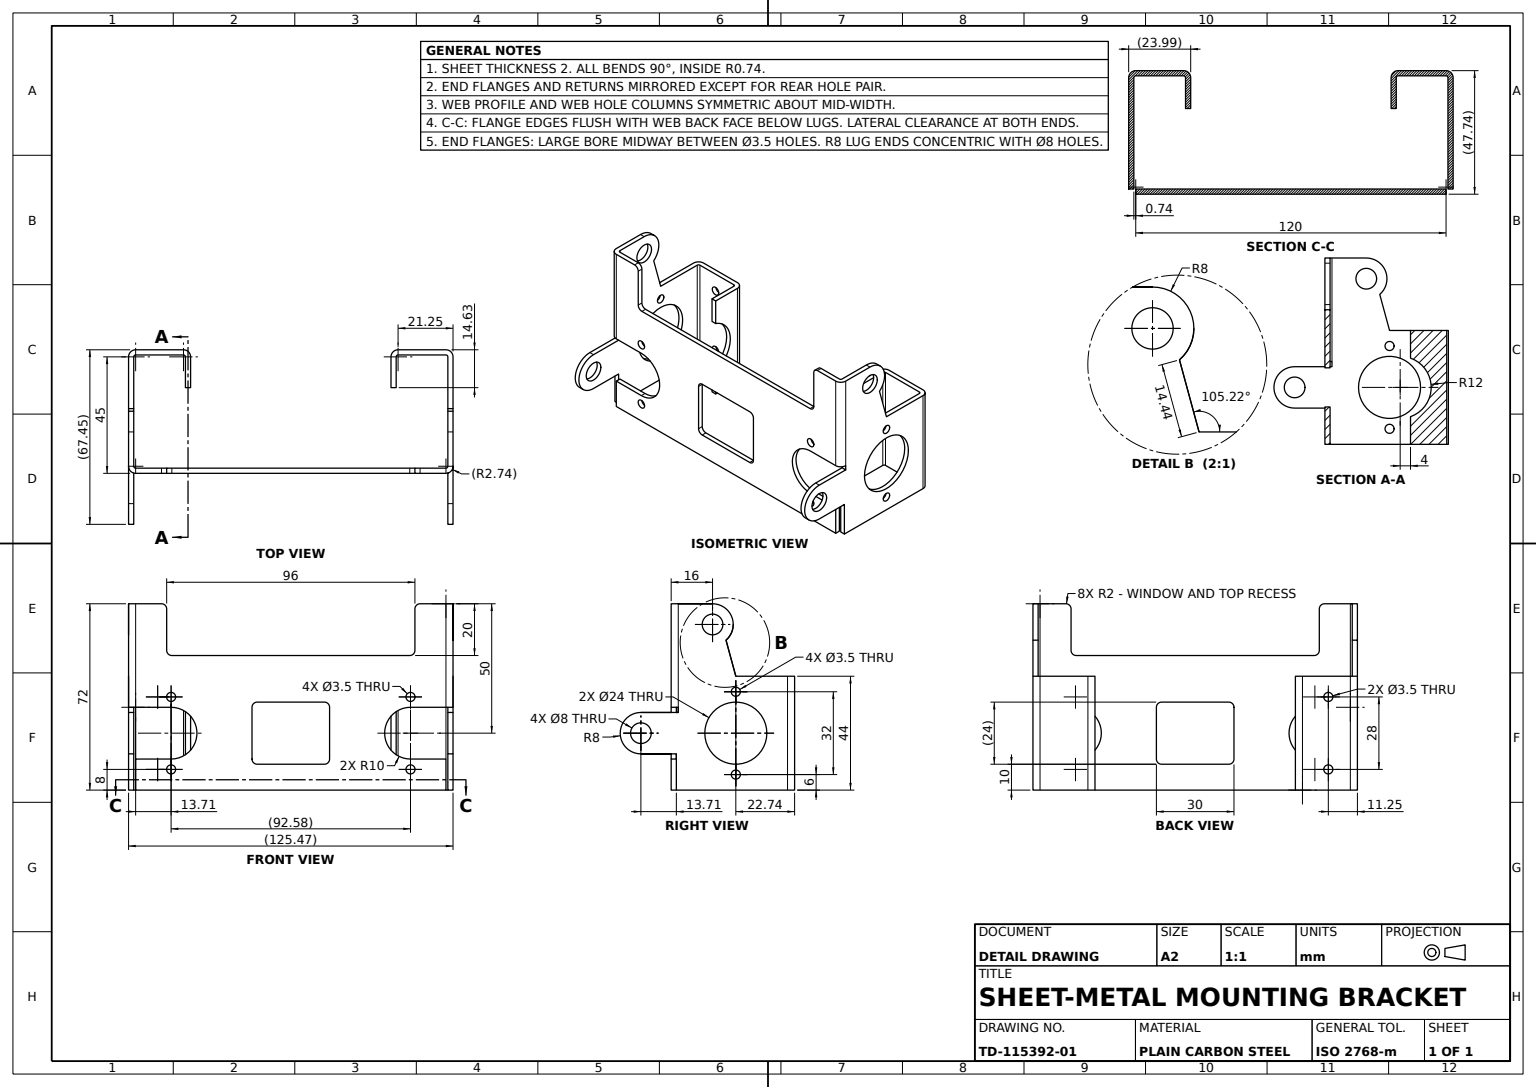
solid
v1 (62.7366,-22,-13.71)
v2 (62.7366,-6,-13.71)
e1 v1 v2 CIRCLE(AX(P(62.7366,-14,-13.71),D(1,0,0),D(0,0,-1)),8)
v3 (60.7366,-22,-13.71)
e2 v1 v3 LINE
v4 (60.7366,-6,-13.71)
e3 v3 v4 CIRCLE(AX(P(60.7366,-14,-13.71),D(1,0,0),D(0,0,-1)),8)
e4 v2 v4 LINE
face CYL(AX(P(62.7366,-14,-13.71),D(-1,0,0),D(0,0,1)),8) [-e1 e2 e3 -e4]
v5 (-46.29,-24,0)
v6 (-60,-24,0)
e5 v5 v6 LINE
v7 (-46.29,-24,-2)
e6 v7 v5 LINE
v8 (-60,-24,-2)
e7 v7 v8 LINE
e8 v8 v6 LINE
face PLANE(AX(P(-46.29,-24,-2),D(0,1,0),D(0,0,1))) [-e5 -e6 e7 e8]
v9 (41.4866,8,45.7366)
v10 (60,8,45.7366)
e9 v9 v10 LINE
v11 (60,8,43.7366)
e10 v11 v10 LINE
v12 (41.4866,8,43.7366)
e11 v12 v11 LINE
e12 v9 v12 LINE
face PLANE(AX(P(60.7366,8,45.7366),D(0,1,0),D(-1,0,0))) [e9 -e10 -e11 -e12]
v13 (60,-4,-2)
v14 (62.7366,-4,0.7366)
e13 v13 v14 CIRCLE(AX(P(60,-4,0.7366),D(0,-1,0),D(0,0,1)),2.7366)
v15 (60,36,-2)
e14 v13 v15 LINE
v16 (62.7366,36,0.7366)
e15 v16 v15 CIRCLE(AX(P(60,36,0.7366),D(0,1,0),D(0,0,1)),2.7366)
e16 v14 v16 LINE
face CYL(AX(P(60,36,0.7366),D(0,1,0),D(1,0,0)),2.7366) [-e13 e14 -e15 -e16]
v17 (60.7366,-30,21.25)
v18 (60.7366,-30,24.75)
e17 v17 v18 CIRCLE(AX(P(60.7366,-30,23),D(1,0,0),D(0,0,-1)),1.75)
e18 v18 v17 CIRCLE(AX(P(60.7366,-30,23),D(1,0,0),D(0,0,-1)),1.75)
v19 (60.7366,-14,-9.71)
v20 (60.7366,-14,-17.71)
e19 v19 v20 CIRCLE(AX(P(60.7366,-14,-13.71),D(1,0,0),D(0,0,-1)),4)
e20 v20 v19 CIRCLE(AX(P(60.7366,-14,-13.71),D(1,0,0),D(0,0,-1)),4)
v21 (60.7366,2,21.25)
v22 (60.7366,2,24.75)
e21 v21 v22 CIRCLE(AX(P(60.7366,2,23),D(1,0,0),D(0,0,-1)),1.75)
e22 v22 v21 CIRCLE(AX(P(60.7366,2,23),D(1,0,0),D(0,0,-1)),1.75)
v23 (60.7366,8,23)
v24 (60.7366,8,43)
e23 v23 v24 LINE
v25 (60.7366,21.93,19.211056)
e24 v25 v23 LINE
v26 (60.7366,28,22)
e25 v26 v25 CIRCLE(AX(P(60.7366,28,14),D(1,0,0),D(0,0,-1)),8)
v27 (60.7366,36,14)
e26 v27 v26 CIRCLE(AX(P(60.7366,28,14),D(1,0,0),D(0,0,-1)),8)
v28 (60.7366,36,0.7366)
e27 v28 v27 LINE
v29 (60.7366,-4,0.7366)
e28 v29 v28 LINE
v30 (60.7366,-6,0.7366)
e29 v30 v29 LINE
e30 v4 v30 LINE
v31 (60.7366,-22,0)
e31 v31 v3 LINE
v32 (60.7366,-36,0)
e32 v32 v31 LINE
v33 (60.7366,-36,43)
e33 v33 v32 LINE
e34 v24 v33 LINE
v34 (60.7366,-14,11)
v35 (60.7366,-14,35)
e35 v34 v35 CIRCLE(AX(P(60.7366,-14,23),D(1,0,0),D(0,0,-1)),12)
e36 v35 v34 CIRCLE(AX(P(60.7366,-14,23),D(1,0,0),D(0,0,-1)),12)
v36 (60.7366,28,18)
v37 (60.7366,28,10)
e37 v36 v37 CIRCLE(AX(P(60.7366,28,14),D(1,0,0),D(0,0,-1)),4)
e38 v37 v36 CIRCLE(AX(P(60.7366,28,14),D(1,0,0),D(0,0,-1)),4)
face PLANE(AX(P(60.7366,28,14),D(1,0,0),D(0,0,-1))) rev [e17 e18] [e19 e20] [e21 e22] [-e23 -e24 -e25 -e26 -e27 -e28 -e29 -e30 -e3 -e31 -e32 -e33 -e34] [e35 e36] [e37 e38]
v38 (-60,8,45.7366)
v39 (-60,-36,45.7366)
e39 v38 v39 LINE
v40 (-41.4866,-36,45.7366)
e40 v39 v40 LINE
v41 (-41.4866,8,45.7366)
e41 v40 v41 LINE
e42 v41 v38 LINE
face PLANE(AX(P(0,0,45.7366),D(0,0,1),D(-1,0,0))) [e39 e40 e41 e42]
v42 (-48.04,0,-2)
v43 (-44.54,0,-2)
e43 v42 v43 CIRCLE(AX(P(-46.29,0,-2),D(0,0,1),D(1,0,0)),1.75)
v44 (-48.04,0,0)
e44 v42 v44 LINE
v45 (-44.54,0,0)
e45 v44 v45 CIRCLE(AX(P(-46.29,0,0),D(0,0,1),D(1,0,0)),1.75)
e46 v43 v45 LINE
face CYL(AX(P(-46.29,0,-2),D(0,0,1),D(1,0,0)),1.75) rev [-e43 e44 e45 -e46]
v46 (-62.7366,-6,-13.71)
v47 (-60.7366,-6,-13.71)
e47 v46 v47 LINE
v48 (-62.7366,-6,0.7366)
e48 v46 v48 LINE
v49 (-60.7366,-6,0.7366)
e49 v49 v48 LINE
e50 v47 v49 LINE
face PLANE(AX(P(-62.7366,-6,-13.71),D(0,1,0),D(-1,0,0))) [-e47 e48 -e49 -e50]
v50 (13,-2,0)
v51 (-13,-2,0)
e51 v50 v51 LINE
v52 (-13,-2,-2)
e52 v52 v51 LINE
v53 (13,-2,-2)
e53 v53 v52 LINE
e54 v53 v50 LINE
face PLANE(AX(P(-13,-2,-2),D(0,1,0),D(-1,0,0))) rev [e51 -e52 -e53 e54]
v54 (62.7366,21.93,19.211056)
e55 v54 v25 LINE
v55 (62.7366,28,22)
e56 v55 v54 CIRCLE(AX(P(62.7366,28,14),D(1,0,0),D(0,0,-1)),8)
e57 v55 v26 LINE
face CYL(AX(P(62.7366,28,14),D(-1,0,0),D(0,0,1)),8) [-e55 -e56 e57 e25]
v56 (-41.4866,8,43.7366)
v57 (-40.75,8,43)
e58 v56 v57 CIRCLE(AX(P(-41.4866,8,43),D(0,1,0),D(0,0,-1)),0.7366)
e59 v41 v56 LINE
v58 (-38.75,8,43)
e60 v41 v58 CIRCLE(AX(P(-41.4866,8,43),D(0,1,0),D(0,0,-1)),2.7366)
e61 v57 v58 LINE
face PLANE(AX(P(-41.4866,8,43),D(0,1,0),D(0,0,1))) [-e58 -e59 e60 -e61]
v59 (49.7366,-28,43.7366)
v60 (49.7366,-28,45.7366)
e62 v59 v60 LINE
v61 (53.2366,-28,45.7366)
e63 v60 v61 CIRCLE(AX(P(51.4866,-28,45.7366),D(0,0,1),D(1,0,0)),1.75)
v62 (53.2366,-28,43.7366)
e64 v62 v61 LINE
e65 v59 v62 CIRCLE(AX(P(51.4866,-28,43.7366),D(0,0,1),D(1,0,0)),1.75)
face CYL(AX(P(51.4866,-28,35.7366),D(0,0,1),D(1,0,0)),1.75) rev [e62 e63 -e64 -e65]
v63 (62.7366,-36,43)
v64 (60,-36,45.7366)
e66 v63 v64 CIRCLE(AX(P(60,-36,43),D(0,-1,0),D(0,0,1)),2.7366)
v65 (62.7366,8,43)
e67 v65 v63 LINE
e68 v10 v65 CIRCLE(AX(P(60,8,43),D(0,1,0),D(0,0,1)),2.7366)
e69 v64 v10 LINE
face CYL(AX(P(60,8,43),D(0,1,0),D(0,0,1)),2.7366) [-e66 -e67 -e68 -e69]
v66 (62.7366,-36,0)
e70 v63 v66 LINE
e71 v63 v33 LINE
e72 v66 v32 LINE
face PLANE(AX(P(62.7366,-36,0),D(0,1,0),D(-1,0,0))) rev [-e70 e71 e33 -e72]
v67 (-62.7366,-22,0)
v68 (-62.7366,-22,-13.71)
e73 v67 v68 LINE
v69 (-60.7366,-22,-13.71)
e74 v68 v69 LINE
v70 (-60.7366,-22,0)
e75 v70 v69 LINE
e76 v67 v70 LINE
face PLANE(AX(P(-62.7366,-22,-13.71),D(0,-1,0),D(1,0,0))) [e73 e74 -e75 -e76]
v71 (40.75,-36,43)
v72 (40.75,-36,31.1066)
e77 v71 v72 LINE
v73 (38.75,-36,43)
e78 v71 v73 LINE
v74 (38.75,-36,31.1066)
e79 v73 v74 LINE
e80 v74 v72 LINE
face PLANE(AX(P(38.75,-36,31.1066),D(0,-1,0),D(1,0,0))) [-e77 e78 e79 e80]
v75 (60,-36,43.7366)
e81 v33 v75 CIRCLE(AX(P(60,-36,43),D(0,-1,0),D(0,0,1)),0.7366)
e82 v75 v11 LINE
e83 v11 v24 CIRCLE(AX(P(60,8,43),D(0,1,0),D(0,0,1)),0.7366)
face CYL(AX(P(60,8,43),D(0,1,0),D(0,0,1)),0.7366) rev [e81 e82 e83 e34]
v76 (62.7366,-22,0)
e84 v76 v1 LINE
e85 v76 v31 LINE
face PLANE(AX(P(62.7366,-22,-13.71),D(0,1,0),D(-1,0,0))) rev [-e2 -e84 e85 e31]
v77 (-38.75,8,31.1066)
e86 v77 v58 LINE
v78 (-40.75,8,31.1066)
e87 v77 v78 LINE
e88 v78 v57 LINE
face PLANE(AX(P(-38.75,8,43.7366),D(0,-1,0),D(1,0,0))) rev [-e86 e87 e88 e61]
v79 (-38.75,-36,43)
e89 v79 v40 CIRCLE(AX(P(-41.4866,-36,43),D(0,-1,0),D(0,0,-1)),2.7366)
e90 v79 v58 LINE
face CYL(AX(P(-41.4866,-36,43),D(0,-1,0),D(1,0,0)),2.7366) [-e60 -e41 -e89 e90]
v80 (-60,-4,-2)
v81 (-46.29,-4,-2)
e91 v80 v81 LINE
v82 (-46.29,-4,0)
e92 v81 v82 LINE
v83 (-60,-4,0)
e93 v83 v82 LINE
e94 v80 v83 LINE
face PLANE(AX(P(-46.29,-4,-2),D(0,-1,0),D(1,0,0))) [e91 e92 -e93 -e94]
v84 (-60.7366,28,10)
v85 (-60.7366,28,18)
e95 v84 v85 CIRCLE(AX(P(-60.7366,28,14),D(1,0,0),D(0,0,1)),4)
v86 (-62.7366,28,18)
e96 v86 v85 LINE
v87 (-62.7366,28,10)
e97 v87 v86 CIRCLE(AX(P(-62.7366,28,14),D(1,0,0),D(0,0,1)),4)
e98 v87 v84 LINE
face CYL(AX(P(-62.7366,28,14),D(1,0,0),D(0,0,-1)),4) rev [e95 -e96 -e97 e98]
v88 (48.04,-28,-2)
v89 (48.04,-28,0)
e99 v88 v89 LINE
v90 (44.54,-28,0)
e100 v89 v90 CIRCLE(AX(P(46.29,-28,0),D(0,0,1),D(-1,0,0)),1.75)
v91 (44.54,-28,-2)
e101 v91 v90 LINE
e102 v88 v91 CIRCLE(AX(P(46.29,-28,-2),D(0,0,1),D(-1,0,0)),1.75)
face CYL(AX(P(46.29,-28,-2),D(0,0,1),D(1,0,0)),1.75) rev [e99 e100 -e101 -e102]
e103 v75 v64 LINE
face PLANE(AX(P(60,-36,43),D(0,-1,0),D(0,0,-1))) [e66 -e103 -e81 -e71]
v92 (62.7366,2,21.25)
v93 (62.7366,2,24.75)
e104 v92 v93 CIRCLE(AX(P(62.7366,2,23),D(1,0,0),D(0,0,-1)),1.75)
e105 v93 v22 LINE
e106 v92 v21 LINE
face CYL(AX(P(62.7366,2,23),D(-1,0,0),D(0,0,1)),1.75) rev [e104 e105 -e21 -e106]
v94 (-62.7366,-4,0.7366)
e107 v94 v48 LINE
v95 (-60.7366,-4,0.7366)
e108 v95 v94 LINE
e109 v95 v49 LINE
face PLANE(AX(P(-60.7366,36,0.7366),D(0,0,-1),D(-1,0,0))) [e49 -e107 -e108 e109]
v96 (41.4866,-36,43.7366)
e110 v96 v71 CIRCLE(AX(P(41.4866,-36,43),D(0,-1,0),D(0,0,1)),0.7366)
v97 (41.4866,-36,45.7366)
e111 v97 v96 LINE
e112 v97 v73 CIRCLE(AX(P(41.4866,-36,43),D(0,-1,0),D(0,0,1)),2.7366)
face PLANE(AX(P(41.4866,-36,43),D(0,-1,0),D(0,0,-1))) [-e78 -e110 -e111 e112]
v98 (62.7366,8,23)
e113 v98 v65 LINE
e114 v98 v23 LINE
e115 v65 v24 LINE
face PLANE(AX(P(62.7366,8,43),D(0,-1,0),D(0,0,-1))) rev [-e113 e114 e23 -e115]
v99 (-60.7366,36,0.7366)
v100 (-62.7366,36,0.7366)
e116 v99 v100 LINE
v101 (-62.7366,36,14)
e117 v100 v101 LINE
v102 (-60.7366,36,14)
e118 v101 v102 LINE
e119 v99 v102 LINE
face PLANE(AX(P(-62.7366,36,14),D(0,1,0),D(-1,0,0))) [e116 e117 e118 -e119]
e120 v29 v14 LINE
v103 (62.7366,-6,0.7366)
e121 v103 v14 LINE
e122 v30 v103 LINE
face PLANE(AX(P(60.7366,-6,0.7366),D(0,0,-1),D(-1,0,0))) [e120 -e121 -e122 e29]
v104 (-38.75,-2.686292,31.1066)
v105 (-40.75,-2.686292,31.1066)
e123 v104 v105 LINE
e124 v105 v78 LINE
e125 v104 v77 LINE
face PLANE(AX(P(-38.75,8,31.1066),D(0,0,1),D(1,0,0))) rev [e123 e124 -e87 -e125]
e126 v100 v94 LINE
v106 (-60,36,-2)
e127 v106 v100 CIRCLE(AX(P(-60,36,0.7366),D(0,1,0),D(0,0,-1)),2.7366)
e128 v106 v80 LINE
e129 v94 v80 CIRCLE(AX(P(-60,-4,0.7366),D(0,-1,0),D(0,0,-1)),2.7366)
face CYL(AX(P(-60,-4,0.7366),D(0,-1,0),D(-1,0,0)),2.7366) [-e126 -e127 e128 -e129]
v107 (-62.7366,2,24.75)
v108 (-60.7366,2,24.75)
e130 v107 v108 LINE
v109 (-60.7366,2,21.25)
e131 v108 v109 CIRCLE(AX(P(-60.7366,2,23),D(1,0,0),D(0,0,1)),1.75)
v110 (-62.7366,2,21.25)
e132 v110 v109 LINE
e133 v107 v110 CIRCLE(AX(P(-62.7366,2,23),D(1,0,0),D(0,0,1)),1.75)
face CYL(AX(P(-62.7366,2,23),D(1,0,0),D(0,0,-1)),1.75) rev [e130 e131 -e132 -e133]
v111 (-15,-4,0)
e134 v51 v111 CIRCLE(AX(P(-13,-4,0),D(0,0,1),D(1,0,0)),2)
v112 (-15,-4,-2)
e135 v112 v111 LINE
e136 v52 v112 CIRCLE(AX(P(-13,-4,-2),D(0,0,1),D(1,0,0)),2)
face CYL(AX(P(-13,-4,-2),D(0,0,1),D(1,0,0)),2) rev [e52 e134 -e135 -e136]
v113 (-62.7366,-36,43)
v114 (-62.7366,-36,0)
e137 v113 v114 LINE
v115 (-60.7366,-36,0)
e138 v114 v115 LINE
v116 (-60.7366,-36,43)
e139 v116 v115 LINE
e140 v113 v116 LINE
face PLANE(AX(P(-62.7366,-36,0),D(0,-1,0),D(1,0,0))) [e137 e138 -e139 -e140]
v117 (-40.75,-36,43)
e141 v117 v79 LINE
v118 (-41.4866,-36,43.7366)
e142 v40 v118 LINE
e143 v117 v118 CIRCLE(AX(P(-41.4866,-36,43),D(0,-1,0),D(0,0,-1)),0.7366)
face PLANE(AX(P(-41.4866,-36,43),D(0,1,0),D(0,0,1))) rev [e141 e89 e142 -e143]
e144 v2 v103 LINE
face PLANE(AX(P(62.7366,-6,-13.71),D(0,-1,0),D(1,0,0))) rev [e4 e30 e122 -e144]
v119 (-60.7366,-14,-9.71)
v120 (-60.7366,-14,-17.71)
e145 v119 v120 CIRCLE(AX(P(-60.7366,-14,-13.71),D(1,0,0),D(0,0,1)),4)
v121 (-62.7366,-14,-17.71)
e146 v121 v120 LINE
v122 (-62.7366,-14,-9.71)
e147 v122 v121 CIRCLE(AX(P(-62.7366,-14,-13.71),D(1,0,0),D(0,0,1)),4)
e148 v122 v119 LINE
face CYL(AX(P(-62.7366,-14,-13.71),D(1,0,0),D(0,0,-1)),4) rev [e145 -e146 -e147 e148]
v123 (50,36,-2)
v124 (48,34,-2)
e149 v123 v124 CIRCLE(AX(P(50,34,-2),D(0,0,1),D(1,0,0)),2)
v125 (48,34,0)
e150 v124 v125 LINE
v126 (50,36,0)
e151 v126 v125 CIRCLE(AX(P(50,34,0),D(0,0,1),D(1,0,0)),2)
e152 v123 v126 LINE
face CYL(AX(P(50,34,-2),D(0,0,1),D(1,0,0)),2) [e149 e150 -e151 -e152]
v127 (-62.7366,21.93,19.211056)
v128 (-60.7366,21.93,19.211056)
e153 v127 v128 LINE
e154 v102 v128 CIRCLE(AX(P(-60.7366,28,14),D(1,0,0),D(0,0,1)),8)
e155 v101 v127 CIRCLE(AX(P(-62.7366,28,14),D(1,0,0),D(0,0,1)),8)
face CYL(AX(P(-62.7366,28,14),D(1,0,0),D(0,0,-1)),8) [e153 -e154 -e118 e155]
v129 (62.7366,36,14)
e156 v129 v27 LINE
e157 v16 v129 LINE
e158 v28 v16 LINE
face PLANE(AX(P(62.7366,36,14),D(0,-1,0),D(1,0,0))) rev [-e156 -e157 -e158 e27]
e159 v86 v87 CIRCLE(AX(P(-62.7366,28,14),D(1,0,0),D(0,0,1)),4)
e160 v85 v84 CIRCLE(AX(P(-60.7366,28,14),D(1,0,0),D(0,0,1)),4)
face CYL(AX(P(-62.7366,28,14),D(1,0,0),D(0,0,-1)),4) rev [-e98 -e159 e96 e160]
v130 (-48.04,-28,0)
v131 (-44.54,-28,0)
e161 v130 v131 CIRCLE(AX(P(-46.29,-28,0),D(0,0,1),D(1,0,0)),1.75)
v132 (-44.54,-28,-2)
e162 v132 v131 LINE
v133 (-48.04,-28,-2)
e163 v133 v132 CIRCLE(AX(P(-46.29,-28,-2),D(0,0,1),D(1,0,0)),1.75)
e164 v133 v130 LINE
face CYL(AX(P(-46.29,-28,-2),D(0,0,1),D(1,0,0)),1.75) rev [e161 -e162 -e163 e164]
v134 (15,-4,-2)
e165 v134 v53 CIRCLE(AX(P(13,-4,-2),D(0,0,1),D(-1,0,0)),2)
v135 (15,-4,0)
e166 v134 v135 LINE
e167 v135 v50 CIRCLE(AX(P(13,-4,0),D(0,0,1),D(-1,0,0)),2)
face CYL(AX(P(13,-4,-2),D(0,0,1),D(1,0,0)),2) rev [-e54 -e165 e166 e167]
v136 (-62.7366,8,23)
v137 (-60.7366,8,23)
e168 v136 v137 LINE
e169 v128 v137 LINE
e170 v127 v136 LINE
face PLANE(AX(P(-62.7366,8,23),D(0,0.262463151,0.964942016),D(0,-0.964942016,0.262463151))) [e168 -e169 -e153 e170]
v138 (-48,18,-2)
v139 (-48,18,0)
e171 v138 v139 LINE
v140 (-48,34,-2)
e172 v138 v140 LINE
v141 (-48,34,0)
e173 v140 v141 LINE
e174 v139 v141 LINE
face PLANE(AX(P(-48,18,-2),D(1,0,0),D(0,0,-1))) [-e171 e172 e173 -e174]
v142 (-60.7366,-14,-21.71)
e175 v142 v47 CIRCLE(AX(P(-60.7366,-14,-13.71),D(1,0,0),D(0,0,1)),8)
v143 (-62.7366,-14,-21.71)
e176 v143 v142 LINE
e177 v143 v46 CIRCLE(AX(P(-62.7366,-14,-13.71),D(1,0,0),D(0,0,1)),8)
face CYL(AX(P(-62.7366,-14,-13.71),D(1,0,0),D(0,0,-1)),8) [e47 -e175 -e176 e177]
e178 v66 v76 LINE
face PLANE(AX(P(62.7366,-36,0),D(0,0,1),D(1,0,0))) rev [e32 -e85 -e178 e72]
e179 v43 v42 CIRCLE(AX(P(-46.29,0,-2),D(0,0,1),D(1,0,0)),1.75)
e180 v45 v44 CIRCLE(AX(P(-46.29,0,0),D(0,0,1),D(1,0,0)),1.75)
face CYL(AX(P(-46.29,0,-2),D(0,0,1),D(1,0,0)),1.75) rev [-e179 e46 e180 -e44]
face PLANE(AX(P(60,8,43),D(0,-1,0),D(0,0,-1))) rev [e68 e115 -e83 e10]
e181 v97 v9 LINE
e182 v64 v97 LINE
v144 (49.7366,0,45.7366)
v145 (53.2366,0,45.7366)
e183 v144 v145 CIRCLE(AX(P(51.4866,0,45.7366),D(0,0,1),D(1,0,0)),1.75)
e184 v145 v144 CIRCLE(AX(P(51.4866,0,45.7366),D(0,0,1),D(1,0,0)),1.75)
e185 v61 v60 CIRCLE(AX(P(51.4866,-28,45.7366),D(0,0,1),D(1,0,0)),1.75)
face PLANE(AX(P(0,0,45.7366),D(0,0,1),D(1,0,0))) [-e181 -e182 e69 -e9] [-e183 -e184] [-e185 -e63]
v146 (46.29,-4,-2)
v147 (46.29,-4,0)
e186 v146 v147 LINE
v148 (46.29,-24,0)
e187 v148 v147 CIRCLE(AX(P(46.29,-14,0),D(0,0,-1),D(1,0,0)),10)
v149 (46.29,-24,-2)
e188 v149 v148 LINE
e189 v149 v146 CIRCLE(AX(P(46.29,-14,-2),D(0,0,-1),D(1,0,0)),10)
face CYL(AX(P(46.29,-14,-2),D(0,0,1),D(1,0,0)),10) rev [e186 -e187 -e188 e189]
e190 v131 v130 CIRCLE(AX(P(-46.29,-28,0),D(0,0,1),D(1,0,0)),1.75)
e191 v132 v133 CIRCLE(AX(P(-46.29,-28,-2),D(0,0,1),D(1,0,0)),1.75)
face CYL(AX(P(-46.29,-28,-2),D(0,0,1),D(1,0,0)),1.75) rev [e190 -e164 -e191 e162]
v150 (49.7366,0,43.7366)
v151 (53.2366,0,43.7366)
e192 v150 v151 CIRCLE(AX(P(51.4866,0,43.7366),D(0,0,1),D(1,0,0)),1.75)
e193 v150 v144 LINE
e194 v151 v145 LINE
face CYL(AX(P(51.4866,0,35.7366),D(0,0,1),D(1,0,0)),1.75) rev [-e192 e193 e183 -e194]
e195 v62 v59 CIRCLE(AX(P(51.4866,-28,43.7366),D(0,0,1),D(1,0,0)),1.75)
face CYL(AX(P(51.4866,-28,35.7366),D(0,0,1),D(1,0,0)),1.75) rev [e185 -e62 -e195 e64]
v152 (-50,36,0)
e196 v141 v152 CIRCLE(AX(P(-50,34,0),D(0,0,1),D(1,0,0)),2)
v153 (-50,36,-2)
e197 v140 v153 CIRCLE(AX(P(-50,34,-2),D(0,0,1),D(1,0,0)),2)
e198 v153 v152 LINE
face CYL(AX(P(-50,34,-2),D(0,0,1),D(1,0,0)),2) [-e196 -e173 e197 e198]
v154 (-40.75,-14,39.1066)
e199 v154 v105 CIRCLE(AX(P(-40.75,-14,27.1066),D(-1,0,0),D(0,0,1)),12)
v155 (-38.75,-14,39.1066)
e200 v155 v104 CIRCLE(AX(P(-38.75,-14,27.1066),D(-1,0,0),D(0,0,1)),12)
e201 v155 v154 LINE
face CYL(AX(P(-38.75,-14,27.1066),D(-1,0,0),D(0,0,1)),12) rev [e199 -e123 -e200 e201]
v156 (48,18,0)
e202 v125 v156 LINE
v157 (48,18,-2)
e203 v124 v157 LINE
e204 v157 v156 LINE
face PLANE(AX(P(48,18,-2),D(-1,0,0),D(0,0,1))) [-e202 -e150 e203 e204]
v158 (-62.7366,-14,35)
v159 (-60.7366,-14,35)
e205 v158 v159 LINE
v160 (-60.7366,-14,11)
e206 v159 v160 CIRCLE(AX(P(-60.7366,-14,23),D(1,0,0),D(0,0,1)),12)
v161 (-62.7366,-14,11)
e207 v161 v160 LINE
e208 v158 v161 CIRCLE(AX(P(-62.7366,-14,23),D(1,0,0),D(0,0,1)),12)
face CYL(AX(P(-62.7366,-14,23),D(1,0,0),D(0,0,-1)),12) rev [e205 e206 -e207 -e208]
v162 (-40.75,-25.313708,31.1066)
e209 v162 v154 CIRCLE(AX(P(-40.75,-14,27.1066),D(-1,0,0),D(0,0,1)),12)
v163 (-38.75,-25.313708,31.1066)
e210 v163 v155 CIRCLE(AX(P(-38.75,-14,27.1066),D(-1,0,0),D(0,0,1)),12)
e211 v163 v162 LINE
face CYL(AX(P(-38.75,-14,27.1066),D(-1,0,0),D(0,0,1)),12) rev [e209 -e201 -e210 e211]
v164 (-38.75,-36,31.1066)
e212 v164 v163 LINE
v165 (-40.75,-36,31.1066)
e213 v164 v165 LINE
e214 v165 v162 LINE
face PLANE(AX(P(-38.75,-25.313708,31.1066),D(0,0,1),D(1,0,0))) rev [-e211 -e212 e213 e214]
v166 (-60,36,0)
e215 v166 v83 LINE
e216 v166 v99 CIRCLE(AX(P(-60,36,0.7366),D(0,1,0),D(0,0,-1)),0.7366)
e217 v99 v95 LINE
e218 v95 v83 CIRCLE(AX(P(-60,-4,0.7366),D(0,-1,0),D(0,0,-1)),0.7366)
face CYL(AX(P(-60,-4,0.7366),D(0,-1,0),D(-1,0,0)),0.7366) rev [-e215 e216 e217 e218]
v167 (62.7366,-30,24.75)
v168 (62.7366,-30,21.25)
e219 v167 v168 CIRCLE(AX(P(62.7366,-30,23),D(1,0,0),D(0,0,-1)),1.75)
e220 v168 v17 LINE
e221 v167 v18 LINE
face CYL(AX(P(62.7366,-30,23),D(-1,0,0),D(0,0,1)),1.75) rev [e219 e220 -e18 -e221]
v169 (-36.29,-14,0)
e222 v169 v5 CIRCLE(AX(P(-46.29,-14,0),D(0,0,-1),D(1,0,0)),10)
v170 (-36.29,-14,-2)
e223 v170 v169 LINE
e224 v170 v7 CIRCLE(AX(P(-46.29,-14,-2),D(0,0,-1),D(1,0,0)),10)
face CYL(AX(P(-46.29,-14,-2),D(0,0,1),D(1,0,0)),10) rev [e6 -e222 -e223 e224]
e225 v110 v107 CIRCLE(AX(P(-62.7366,2,23),D(1,0,0),D(0,0,1)),1.75)
e226 v109 v108 CIRCLE(AX(P(-60.7366,2,23),D(1,0,0),D(0,0,1)),1.75)
face CYL(AX(P(-62.7366,2,23),D(1,0,0),D(0,0,-1)),1.75) rev [-e130 -e225 e132 e226]
v171 (38.75,-2.686292,31.1066)
v172 (38.75,8,31.1066)
e227 v171 v172 LINE
v173 (38.75,-25.313708,31.1066)
e228 v173 v171 CIRCLE(AX(P(38.75,-14,27.1066),D(-1,0,0),D(0,0,-1)),12)
e229 v74 v173 LINE
v174 (38.75,8,43)
e230 v174 v73 LINE
e231 v172 v174 LINE
face PLANE(AX(P(38.75,-14,27.1066),D(1,0,0),D(0,0,-1))) rev [-e227 -e228 -e229 -e79 -e230 -e231]
e232 v117 v165 LINE
e233 v79 v164 LINE
face PLANE(AX(P(-38.75,-36,31.1066),D(0,1,0),D(-1,0,0))) rev [e232 -e213 -e233 -e141]
v175 (-15,-24,-2)
v176 (-15,-24,0)
e234 v175 v176 LINE
e235 v112 v175 LINE
e236 v111 v176 LINE
face PLANE(AX(P(-15,-4,-2),D(-1,0,0),D(0,-1,0))) rev [-e234 -e235 e135 e236]
v177 (62.7366,-14,-9.71)
e237 v177 v19 LINE
v178 (62.7366,-14,-17.71)
e238 v177 v178 CIRCLE(AX(P(62.7366,-14,-13.71),D(1,0,0),D(0,0,-1)),4)
e239 v178 v20 LINE
face CYL(AX(P(62.7366,-14,-13.71),D(-1,0,0),D(0,0,1)),4) rev [-e19 -e237 e238 e239]
v179 (62.7366,-14,11)
e240 v179 v34 LINE
v180 (62.7366,-14,35)
e241 v179 v180 CIRCLE(AX(P(62.7366,-14,23),D(1,0,0),D(0,0,-1)),12)
e242 v180 v35 LINE
face CYL(AX(P(62.7366,-14,23),D(-1,0,0),D(0,0,1)),12) rev [-e240 e241 e242 -e35]
v181 (-60,-36,43.7366)
e243 v181 v118 LINE
e244 v181 v39 LINE
face PLANE(AX(P(-41.4866,-36,45.7366),D(0,1,0),D(-1,0,0))) rev [e243 -e142 -e40 -e244]
v182 (40.75,8,43)
e245 v182 v12 CIRCLE(AX(P(41.4866,8,43),D(0,1,0),D(0,0,1)),0.7366)
e246 v96 v12 LINE
e247 v71 v182 LINE
face CYL(AX(P(41.4866,8,43),D(0,1,0),D(-1,0,0)),0.7366) rev [e245 -e246 e110 e247]
v183 (62.7366,28,10)
v184 (62.7366,28,18)
e248 v183 v184 CIRCLE(AX(P(62.7366,28,14),D(1,0,0),D(0,0,-1)),4)
e249 v184 v36 LINE
e250 v183 v37 LINE
face CYL(AX(P(62.7366,28,14),D(-1,0,0),D(0,0,1)),4) rev [e248 e249 -e38 -e250]
v185 (60,-36,-2)
v186 (60,-36,0)
e251 v185 v186 LINE
v187 (-60,-36,0)
e252 v187 v186 LINE
v188 (-60,-36,-2)
e253 v188 v187 LINE
e254 v188 v185 LINE
face PLANE(AX(P(-60,-36,-2),D(0,-1,0),D(0,0,-1))) [e251 -e252 -e253 e254]
v189 (60,36,0)
e255 v15 v189 LINE
e256 v28 v189 CIRCLE(AX(P(60,36,0.7366),D(0,1,0),D(0,0,1)),0.7366)
face PLANE(AX(P(60,36,0.7366),D(0,-1,0),D(0,0,-1))) rev [e255 -e256 e158 e15]
e257 v160 v159 CIRCLE(AX(P(-60.7366,-14,23),D(1,0,0),D(0,0,1)),12)
v190 (-60.7366,-30,24.75)
v191 (-60.7366,-30,21.25)
e258 v190 v191 CIRCLE(AX(P(-60.7366,-30,23),D(1,0,0),D(0,0,1)),1.75)
e259 v191 v190 CIRCLE(AX(P(-60.7366,-30,23),D(1,0,0),D(0,0,1)),1.75)
e260 v115 v70 LINE
e261 v69 v142 CIRCLE(AX(P(-60.7366,-14,-13.71),D(1,0,0),D(0,0,1)),8)
v192 (-60.7366,8,43)
e262 v137 v192 LINE
e263 v192 v116 LINE
e264 v120 v119 CIRCLE(AX(P(-60.7366,-14,-13.71),D(1,0,0),D(0,0,1)),4)
face PLANE(AX(P(-60.7366,28,14),D(-1,0,0),D(0,0,-1))) rev [-e257 -e206] [-e258 -e259] [-e131 -e226] [e260 e75 e261 e175 e50 -e109 -e217 e119 e154 e169 e262 e263 e139] [-e264 -e145] [-e160 -e95]
v193 (60,-4,0)
e265 v193 v29 CIRCLE(AX(P(60,-4,0.7366),D(0,-1,0),D(0,0,1)),0.7366)
e266 v13 v193 LINE
face PLANE(AX(P(60,-4,0.7366),D(0,-1,0),D(0,0,-1))) [e13 -e120 -e265 -e266]
e267 v153 v106 LINE
e268 v106 v166 LINE
e269 v152 v166 LINE
face PLANE(AX(P(-60,36,-2),D(0,1,0),D(0,0,1))) [-e198 e267 e268 -e269]
e270 v178 v177 CIRCLE(AX(P(62.7366,-14,-13.71),D(1,0,0),D(0,0,-1)),4)
face CYL(AX(P(62.7366,-14,-13.71),D(-1,0,0),D(0,0,1)),4) rev [-e239 e270 e237 -e20]
e271 v146 v13 LINE
e272 v147 v193 LINE
face PLANE(AX(P(46.29,-4,-2),D(0,-1,0),D(0,0,-1))) [e271 e266 -e272 -e186]
v194 (15,-24,0)
e273 v194 v135 LINE
v195 (15,-24,-2)
e274 v195 v134 LINE
e275 v195 v194 LINE
face PLANE(AX(P(15,-4,-2),D(1,0,0),D(0,1,0))) rev [e273 -e166 -e274 e275]
e276 v129 v55 CIRCLE(AX(P(62.7366,28,14),D(1,0,0),D(0,0,-1)),8)
face CYL(AX(P(62.7366,28,14),D(-1,0,0),D(0,0,1)),8) [e156 e26 -e57 -e276]
v196 (-62.7366,8,43)
e277 v196 v192 LINE
e278 v136 v196 LINE
face PLANE(AX(P(-62.7366,8,43),D(0,1,0),D(0,0,1))) [e277 -e262 -e168 e278]
e279 v121 v122 CIRCLE(AX(P(-62.7366,-14,-13.71),D(1,0,0),D(0,0,1)),4)
face CYL(AX(P(-62.7366,-14,-13.71),D(1,0,0),D(0,0,-1)),4) rev [-e279 e146 e264 -e148]
v197 (46,16,0)
e280 v156 v197 CIRCLE(AX(P(46,18,0),D(0,0,-1),D(1,0,0)),2)
v198 (46,16,-2)
e281 v157 v198 CIRCLE(AX(P(46,18,-2),D(0,0,-1),D(1,0,0)),2)
e282 v198 v197 LINE
face CYL(AX(P(46,18,-2),D(0,0,1),D(1,0,0)),2) rev [-e280 -e204 e281 e282]
v199 (-62.7366,-30,21.25)
v200 (-62.7366,-30,24.75)
e283 v199 v200 CIRCLE(AX(P(-62.7366,-30,23),D(1,0,0),D(0,0,1)),1.75)
e284 v200 v199 CIRCLE(AX(P(-62.7366,-30,23),D(1,0,0),D(0,0,1)),1.75)
e285 v161 v158 CIRCLE(AX(P(-62.7366,-14,23),D(1,0,0),D(0,0,1)),12)
e286 v196 v113 LINE
e287 v68 v143 CIRCLE(AX(P(-62.7366,-14,-13.71),D(1,0,0),D(0,0,1)),8)
e288 v114 v67 LINE
face PLANE(AX(P(-62.7366,28,14),D(-1,0,0),D(0,0,-1))) [e159 e97] [e283 e284] [e225 e133] [e208 e285] [e279 e147] [-e137 -e286 -e278 -e170 -e155 -e117 e126 e107 -e48 -e177 -e287 -e73 -e288]
e289 v93 v92 CIRCLE(AX(P(62.7366,2,23),D(1,0,0),D(0,0,-1)),1.75)
face CYL(AX(P(62.7366,2,23),D(-1,0,0),D(0,0,1)),1.75) rev [-e105 e289 e106 -e22]
e290 v200 v190 LINE
e291 v199 v191 LINE
face CYL(AX(P(-62.7366,-30,23),D(1,0,0),D(0,0,-1)),1.75) rev [-e290 -e283 e291 e259]
e292 v39 v113 CIRCLE(AX(P(-60,-36,43),D(0,-1,0),D(0,0,-1)),2.7366)
e293 v181 v116 CIRCLE(AX(P(-60,-36,43),D(0,-1,0),D(0,0,-1)),0.7366)
face PLANE(AX(P(-60,-36,43),D(0,1,0),D(0,0,1))) rev [e292 e140 -e293 e244]
v201 (-46,16,0)
e294 v201 v139 CIRCLE(AX(P(-46,18,0),D(0,0,-1),D(-1,0,0)),2)
v202 (-46,16,-2)
e295 v202 v201 LINE
e296 v202 v138 CIRCLE(AX(P(-46,18,-2),D(0,0,-1),D(-1,0,0)),2)
face CYL(AX(P(-46,18,-2),D(0,0,1),D(1,0,0)),2) rev [-e294 -e295 e296 e171]
v203 (-60,8,43.7366)
e297 v192 v203 CIRCLE(AX(P(-60,8,43),D(0,1,0),D(0,0,-1)),0.7366)
e298 v203 v181 LINE
face CYL(AX(P(-60,-36,43),D(0,-1,0),D(0,0,1)),0.7366) rev [-e263 e297 e298 e293]
face PLANE(AX(P(-62.7366,-36,0),D(0,0,-1),D(-1,0,0))) [-e138 e288 e76 -e260]
e299 v90 v89 CIRCLE(AX(P(46.29,-28,0),D(0,0,1),D(-1,0,0)),1.75)
e300 v91 v88 CIRCLE(AX(P(46.29,-28,-2),D(0,0,1),D(-1,0,0)),1.75)
face CYL(AX(P(46.29,-28,-2),D(0,0,1),D(1,0,0)),1.75) rev [e299 -e99 -e300 e101]
e301 v81 v170 CIRCLE(AX(P(-46.29,-14,-2),D(0,0,-1),D(1,0,0)),10)
e302 v82 v169 CIRCLE(AX(P(-46.29,-14,0),D(0,0,-1),D(1,0,0)),10)
face CYL(AX(P(-46.29,-14,-2),D(0,0,1),D(1,0,0)),10) rev [-e92 e301 e223 -e302]
e303 v198 v202 LINE
e304 v197 v201 LINE
face PLANE(AX(P(-46,16,-2),D(0,1,0),D(0,0,1))) [-e282 e303 e295 -e304]
e305 v196 v38 CIRCLE(AX(P(-60,8,43),D(0,1,0),D(0,0,-1)),2.7366)
face CYL(AX(P(-60,-36,43),D(0,-1,0),D(0,0,1)),2.7366) [e286 -e292 -e39 -e305]
e306 v15 v123 LINE
e307 v189 v126 LINE
face PLANE(AX(P(50,36,-2),D(0,1,0),D(0,0,1))) [-e255 e306 e152 -e307]
e308 v151 v150 CIRCLE(AX(P(51.4866,0,43.7366),D(0,0,1),D(1,0,0)),1.75)
e309 v75 v96 LINE
face PLANE(AX(P(0,0,43.7366),D(0,0,1),D(1,0,0))) rev [e192 e308] [e195 e65] [-e82 e309 e246 e11]
e310 v56 v203 LINE
e311 v118 v56 LINE
face PLANE(AX(P(0,0,43.7366),D(0,0,1),D(-1,0,0))) rev [-e298 -e310 -e311 -e243]
v204 (13,-26,-2)
e312 v204 v195 CIRCLE(AX(P(13,-24,-2),D(0,0,1),D(1,0,0)),2)
v205 (-13,-26,-2)
e313 v175 v205 CIRCLE(AX(P(-13,-24,-2),D(0,0,1),D(1,0,0)),2)
e314 v205 v204 LINE
v206 (60,-24,-2)
e315 v206 v149 LINE
e316 v185 v206 LINE
e317 v8 v188 LINE
v207 (44.54,0,-2)
v208 (48.04,0,-2)
e318 v207 v208 CIRCLE(AX(P(46.29,0,-2),D(0,0,1),D(-1,0,0)),1.75)
e319 v208 v207 CIRCLE(AX(P(46.29,0,-2),D(0,0,1),D(-1,0,0)),1.75)
face PLANE(AX(P(-46.29,-14,-2),D(0,0,1),D(1,0,0))) rev [e43 e179] [e102 e300] [e312 e274 e165 e53 e136 e235 e313 e314] [-e306 -e14 -e271 -e189 -e315 -e316 -e254 -e317 -e7 -e224 -e301 -e91 -e128 -e267 -e197 -e172 -e296 -e303 -e281 -e203 -e149] [e318 e319] [e191 e163]
v209 (60,-24,0)
e320 v186 v209 LINE
e321 v206 v209 LINE
face PLANE(AX(P(60,-24,-2),D(1,0,0),D(0,1,0))) [-e320 -e251 e316 e321]
v210 (44.54,0,0)
v211 (48.04,0,0)
e322 v210 v211 CIRCLE(AX(P(46.29,0,0),D(0,0,1),D(-1,0,0)),1.75)
e323 v208 v211 LINE
e324 v207 v210 LINE
face CYL(AX(P(46.29,0,-2),D(0,0,1),D(1,0,0)),1.75) rev [e322 -e323 -e318 e324]
face PLANE(AX(P(-60,-4,0.7366),D(0,1,0),D(0,0,1))) rev [e108 e129 e94 -e218]
v212 (-13,-26,0)
e325 v176 v212 CIRCLE(AX(P(-13,-24,0),D(0,0,1),D(1,0,0)),2)
e326 v205 v212 LINE
face CYL(AX(P(-13,-24,-2),D(0,0,1),D(1,0,0)),2) rev [e234 e325 -e326 -e313]
e327 v57 v117 LINE
face CYL(AX(P(-41.4866,-36,43),D(0,-1,0),D(1,0,0)),0.7366) rev [e311 e58 e327 e143]
v213 (40.75,-25.313708,31.1066)
v214 (40.75,-2.686292,31.1066)
e328 v213 v214 CIRCLE(AX(P(40.75,-14,27.1066),D(-1,0,0),D(0,0,-1)),12)
e329 v173 v213 LINE
e330 v171 v214 LINE
face CYL(AX(P(38.75,-14,27.1066),D(1,0,0),D(0,0,-1)),12) rev [-e328 -e329 e228 e330]
face PLANE(AX(P(-60,36,0.7366),D(0,1,0),D(0,0,1))) [-e268 e127 -e116 -e216]
e331 v174 v9 CIRCLE(AX(P(41.4866,8,43),D(0,1,0),D(0,0,1)),2.7366)
face CYL(AX(P(41.4866,8,43),D(0,1,0),D(-1,0,0)),2.7366) [e230 -e112 e181 -e331]
e332 v180 v179 CIRCLE(AX(P(62.7366,-14,23),D(1,0,0),D(0,0,-1)),12)
face CYL(AX(P(62.7366,-14,23),D(-1,0,0),D(0,0,1)),12) rev [e332 e240 -e36 -e242]
e333 v209 v148 LINE
face PLANE(AX(P(46.29,-24,-2),D(0,1,0),D(0,0,1))) [e188 -e333 -e321 e315]
e334 v203 v38 LINE
face PLANE(AX(P(-60,8,43),D(0,1,0),D(0,0,1))) [-e334 -e297 -e277 e305]
v215 (13,-26,0)
e335 v204 v215 LINE
e336 v215 v194 CIRCLE(AX(P(13,-24,0),D(0,0,1),D(1,0,0)),2)
face CYL(AX(P(13,-24,-2),D(0,0,1),D(1,0,0)),2) rev [-e275 -e312 e335 e336]
e337 v6 v187 LINE
face PLANE(AX(P(-60,-24,-2),D(-1,0,0),D(0,-1,0))) [e253 -e337 -e8 e317]
e338 v72 v213 LINE
face PLANE(AX(P(38.75,-25.313708,31.1066),D(0,0,-1),D(-1,0,0))) [e229 e329 -e338 -e80]
face PLANE(AX(P(-38.75,-14,27.1066),D(-1,0,0),D(0,0,-1))) rev [e200 e125 e86 -e90 e233 e212 e210]
e339 v212 v215 LINE
face PLANE(AX(P(-13,-26,-2),D(0,-1,0),D(0,0,-1))) rev [-e335 -e314 e326 e339]
e340 v168 v167 CIRCLE(AX(P(62.7366,-30,23),D(1,0,0),D(0,0,-1)),1.75)
face CYL(AX(P(62.7366,-30,23),D(-1,0,0),D(0,0,1)),1.75) rev [-e17 -e220 e340 e221]
face CYL(AX(P(-62.7366,-30,23),D(1,0,0),D(0,0,-1)),1.75) rev [-e291 -e284 e290 e258]
face PLANE(AX(P(41.4866,-36,45.7366),D(0,-1,0),D(1,0,0))) [e111 -e309 e103 e182]
v216 (40.75,8,31.1066)
e341 v172 v216 LINE
e342 v182 v174 LINE
e343 v216 v182 LINE
face PLANE(AX(P(38.75,8,43.7366),D(0,1,0),D(-1,0,0))) [-e341 e231 -e342 -e343]
face CYL(AX(P(-62.7366,-14,-13.71),D(1,0,0),D(0,0,-1)),8) [e287 e176 -e261 -e74]
e344 v184 v183 CIRCLE(AX(P(62.7366,28,14),D(1,0,0),D(0,0,-1)),4)
e345 v54 v98 LINE
face PLANE(AX(P(62.7366,28,14),D(1,0,0),D(0,0,-1))) [-e248 -e344] [-e241 -e332] [-e340 -e219] [-e270 -e238] [e1 e144 e121 e16 e157 e276 e56 e345 e113 e67 e70 e178 e84] [-e104 -e289]
face CYL(AX(P(-62.7366,-14,23),D(1,0,0),D(0,0,-1)),12) rev [e207 e257 -e205 -e285]
e346 v193 v189 LINE
face CYL(AX(P(60,36,0.7366),D(0,1,0),D(1,0,0)),0.7366) rev [-e346 e265 e28 e256]
e347 v211 v210 CIRCLE(AX(P(46.29,0,0),D(0,0,1),D(-1,0,0)),1.75)
face PLANE(AX(P(-46.29,-14,0),D(0,0,1),D(1,0,0))) [-e100 -e299] [-e190 -e161] [e346 e307 e151 e202 e280 e304 e294 e174 e196 e269 e215 e93 e302 e222 e5 e337 e252 e320 e333 e187 e272] [-e322 -e347] [-e325 -e236 -e134 -e51 -e167 -e273 -e336 -e339] [-e180 -e45]
face PLANE(AX(P(62.7366,8,23),D(0,-0.262463151,-0.964942016),D(0,0.964942016,-0.262463151))) rev [e55 e24 -e114 -e345]
face CYL(AX(P(51.4866,0,35.7366),D(0,0,1),D(1,0,0)),1.75) rev [-e308 e194 e184 -e193]
face CYL(AX(P(46.29,0,-2),D(0,0,1),D(1,0,0)),1.75) rev [-e324 -e319 e323 e347]
face CYL(AX(P(62.7366,28,14),D(-1,0,0),D(0,0,1)),4) rev [e344 e250 -e37 -e249]
e348 v214 v216 LINE
face PLANE(AX(P(38.75,8,31.1066),D(0,0,-1),D(-1,0,0))) [-e330 e227 e341 -e348]
face PLANE(AX(P(-60.7366,8,45.7366),D(0,-1,0),D(1,0,0))) rev [-e42 e59 e310 e334]
face PLANE(AX(P(41.4866,8,43),D(0,-1,0),D(0,0,-1))) rev [e12 -e245 e342 e331]
face PLANE(AX(P(40.75,-14,27.1066),D(1,0,0),D(0,0,-1))) [e348 e343 -e247 e77 e338 e328]
face PLANE(AX(P(-40.75,-14,27.1066),D(-1,0,0),D(0,0,-1))) [-e327 -e88 -e124 -e199 -e209 -e214 -e232]
